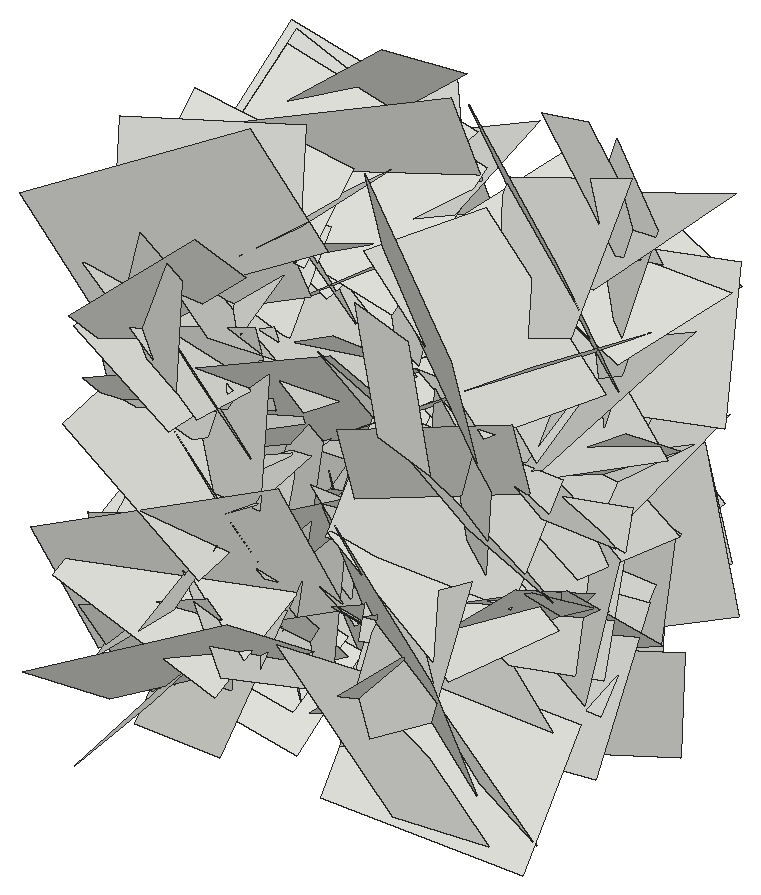
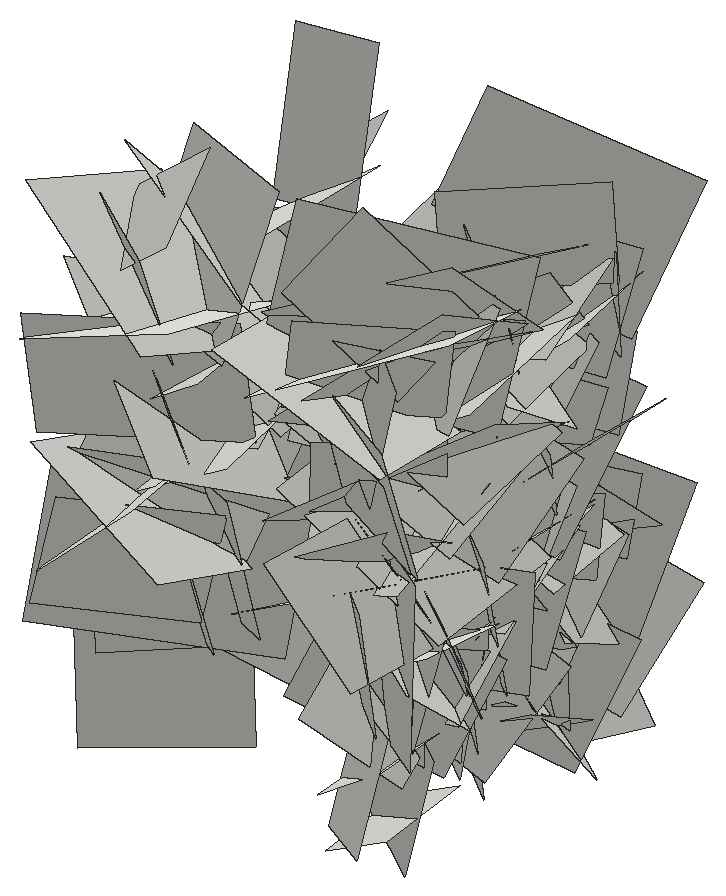
# SketchUp Ruby script. Lengths in inches.
U = 1.inch
M = Sketchup.active_model
def pt(a) = Geom::Point3d.new(a.map { |v| v * U })
def face(e, loops, mat)
  f = e.add_face(loops[0].map { |a| pt(a) })
  loops[1..].each { |l| e.add_face(l.map { |a| pt(a) }).erase! }
  f.material = f.back_material = mat if mat
  f
end
# faces: each face lists its corners as indices into pts; further lists are holes
def faces(e, pts, list, mat = nil) = list.each { |f| face(e, (f[0].is_a?(Array) ? f : [f]).map { |l| l.map { |i| pts[i] } }, mat) }
# xy, xz, yz: faces in a plane at the given z, y or x. An outline is a flat list of corners, or four numbers for a rectangle; further outlines are holes
def ring(l) = l.size == 4 ? [[l[0], l[1]], [l[2], l[1]], [l[2], l[3]], [l[0], l[3]]] : l.each_slice(2).to_a
def flat(e, list, mat, &to3) = list.each { |f| face(e, (f[0].is_a?(Array) ? f : [f]).map { |l| ring(l).map { |u, v| to3.(u, v) } }, mat) }
def xy(e, z, list, mat = nil) = flat(e, list, mat) { |x, y| [x, y, z] }
def xz(e, y, list, mat = nil) = flat(e, list, mat) { |x, z| [x, y, z] }
def yz(e, x, list, mat = nil) = flat(e, list, mat) { |y, z| [x, y, z] }
def lines(e, pts, list) = list.each { |a, b| e.add_line(pt(pts[a]), pt(pts[b])) }
# prism: a flat outline (further loops are holes) pulled along v
def prism(e, loops, v, mat = nil)
  f = face(e, loops, mat); d = Geom::Vector3d.new(v.map { |x| x * U })
  f.pushpull(f.normal.samedirection?(d) ? d.length : -d.length)
end
def box(e, o, s, mat = nil) = prism(e, [[o, [o[0] + s[0], o[1], o[2]], [o[0] + s[0], o[1] + s[1], o[2]], [o[0], o[1] + s[1], o[2]]]], [0, 0, s[2]], mat)
def at(x, y, z, deg = 0) = Geom::Transformation.translation(pt([x, y, z])) * Geom::Transformation.rotation(ORIGIN, Z_AXIS, deg.degrees)
def axes(o, x, y, z) = Geom::Transformation.new([*x, 0, *y, 0, *z, 0, *pt(o).to_a, 1])
def part(name) = M.definitions.add(name)
# library, detail: a bought-in or finely detailed component or shape, given as its bounding box
def library(name, o, s) = part(name).tap { |d| box(d.entities, o, s) }
def detail(e, o, s) = box(e.add_group.entities, o, s)
def put(e, d, t, mat = nil) = e.add_instance(d, t).tap { |i| i.material = mat if mat }
def group(e, t, mat = nil) = e.add_group.tap { |g| g.transformation = t; g.material = mat if mat }.entities
root = M.entities
c1 = part("Component\#6")
p = [[0.01,0,0],[0,3.24,4.54],[4.32,3.24,4.54],[4.33,0,0]]
faces(c1.entities,p,[[0,1,2,3]])
put(root,c1,axes([414.68,153.18,27.99],[0.08911,-1.01671,-0.11332],[0.1646,-0.0997,1.00972],[-1.07181,-0.09984,0.14565]))
put(root,c1,axes([410.71,160.42,26.72],[-0.04031,-0.6417,-0.5437],[0.04231,-0.54502,0.64047],[0.89052,-0.00315,-0.05504]))
put(root,c1,axes([414.68,152.86,32.22],[0.07765,-0.95123,0.12327],[0.10469,0.13045,0.94796],[-1.01133,-0.05954,0.1076]))
put(root,c1,axes([414.68,152.23,36.27],[-0.17612,0.33723,0.58016],[0.03508,0.60107,-0.33991],[-0.71045,-0.05392,-0.16061]))
put(root,c1,axes([410.71,156.02,27.27],[0.01737,0.78195,0.05447],[0.0729,0.05284,-0.77921],[0.82768,-0.02106,0.06749]))
put(root,c1,axes([410.71,151.43,29.49],[-0.01376,0.93036,0.01045],[-0.09599,0.00914,-0.92605],[0.98156,0.01394,-0.09041]))
put(root,c1,axes([410.71,155.63,34.51],[-0.04715,-0.7148,-0.47013],[0.06325,-0.47221,0.71232],[0.90467,-0.00424,-0.0743]))
put(root,c1,axes([414.68,159.35,19.53],[-0.12506,-0.65018,0.20227],[0.00025,0.20525,0.65988],[-0.72178,0.11273,-0.03482]))
put(root,c1,axes([414.68,154.14,39.875],[0.07687,-0.17009,-0.90128],[0.07958,-0.89996,0.17589],[-0.96896,-0.0874,-0.05706]))
put(root,c1,axes([410.71,161.57,34.4],[-0.05292,-0.24359,-0.78611],[0.1523,-0.77804,0.23197],[0.85897,0.12294,-0.08956]))
put(root,c1,axes([410.71,150.44,37.52],[-0.01758,-0.03984,-0.83316],[0.08726,-0.82933,0.03802],[0.87984,0.08145,-0.02042]))
put(root,c1,axes([410.71,152.86,25.21],[0.07237,-0.84668,-0.40971],[-0.16913,-0.41526,0.83156],[0.98259,-0.00911,0.17331]))
put(root,c1,axes([410.71,151.53,22],[-0.08087,0.78957,0.40941],[0.10212,0.41583,-0.78401],[0.93722,0.02282,0.12075]))
put(root,c1,axes([410.71,158.82,28.52],[-0.0834,-0.34729,-0.88838],[0.00654,-0.89156,0.34799],[1.01106,-0.02288,-0.07553]))
put(root,c1,axes([414.68,156.05,22.34],[-0.04217,-0.56806,-0.37659],[-0.07293,-0.37196,0.56834],[-0.71876,0.07107,-0.03557]))
put(root,c1,axes([414.68,160.84,30.26],[-0.09118,-0.56201,-0.30691],[-0.0596,-0.30185,0.56849],[-0.67615,0.1024,-0.00872]))
put(root,c1,axes([410.71,154.61,36.92],[-0.07328,1.03426,0.55463],[-0.26621,0.52968,-1.01904],[1.21518,0.17841,-0.1898]))
put(root,c1,axes([414.68,159.76,21.63],[-0.09665,-0.666,0.12875],[0.03078,0.12595,0.67212],[-0.71837,0.095,0.01147]))
put(root,c1,axes([414.68,147.16,24.1],[0.03025,0.92414,0.23442],[0.23339,0.2218,-0.90118],[-0.98329,0.08108,-0.20669]))
put(root,c1,axes([410.71,157.73,31.39],[-0.13129,-0.92283,0.37392],[0.04334,0.37177,0.93107],[1.05456,-0.13017,0.00829]))
put(root,c1,axes([414.68,159.1875,20.3125],[0.01409,-0.35632,0.80543],[0.16766,0.79339,0.34838],[-0.91839,0.13938,0.07596]))
put(root,c1,axes([414.68,153.92,21.15],[0.0271,-0.2919,0.8704],[0.20523,0.85287,0.28034],[-0.95124,0.17569,0.08528]))
put(root,c1,axes([414.68,149.63,26.39],[0.05575,0.3601,-0.58557],[-0.15834,-0.56726,-0.36226],[-0.71127,0.15451,0.03475]))
put(root,c1,axes([414.68,150.69,21.46],[0.08617,-0.06424,0.73191],[-0.1147,0.7273,0.07585],[-0.77031,-0.11548,0.07058]))
put(root,c1,axes([410.71,152.31,24.83],[0.14132,0.38772,0.61473],[0.11706,0.60692,-0.40674],[0.76145,-0.16526,-0.05156]))
put(root,c1,axes([410.71,150.4,30.92],[0.04252,-0.27759,0.76161],[0.13298,0.75548,0.26875],[0.84891,-0.10444,-0.08025]))
put(root,c1,axes([414.68,156.49,28.09],[-0.01227,0.36562,0.53928],[-0.0952,0.53332,-0.36351],[-0.68404,-0.08079,0.04092]))
put(root,c1,axes([410.71,150.56,37.37],[0.01495,0.72639,-0.4873],[0.06872,-0.48689,-0.7239],[0.92463,0.02444,0.06168]))
put(root,c1,axes([414.68,156.34,37.48],[0.20366,-0.78098,-0.33642],[-0.07649,-0.35863,0.79133],[-0.89812,-0.14656,-0.14368]))
put(root,c1,axes([410.71,156.72,22.08],[-0.00521,-0.94479,0.50901],[-0.17637,0.50353,0.93301],[1.12382,0.07464,0.14878]))
put(root,c1,axes([414.68,158.75,26.14],[-0.12859,0.59437,-0.23179],[0.06253,-0.22448,-0.60651],[-0.67335,-0.13435,-0.01206]))
put(root,c1,axes([410.71,154.45,36.57],[0.07713,0.81709,0.22722],[0.03645,0.22503,-0.82021],[0.89825,-0.07929,0.01378]))
put(root,c1,axes([414.68,149.71,29.1],[-0.04042,0.22115,-0.567],[-0.10046,-0.56334,-0.21335],[-0.63725,0.07479,0.0696]))
put(root,c1,axes([414.68,153.82,25.23],[-0.04726,-0.11023,0.59197],[-0.093,0.58845,0.10297],[-0.63147,-0.07841,-0.05947]))
put(root,c1,axes([410.71,150.92,33.45],[-0.01124,-0.40239,0.85237],[0.02564,0.85203,0.40253],[0.99881,-0.0264,-0.00074]))
put(root,c1,axes([410.71,152.27,30.34],[0.04267,0.47891,-0.74389],[0.05776,-0.74459,-0.47642],[0.93603,0.02411,0.06331]))
put(root,c1,axes([410.71,153.79,24.7],[-0.00565,-0.43188,0.90191],[-0.04751,0.90112,0.43124],[1.05892,0.03812,0.02416]))
put(root,c1,axes([410.71,160.9375,37.33],[0.13153,0.12633,-0.90974],[-0.10231,-0.91113,-0.13969],[0.96819,-0.11344,0.10882]))
put(root,c1,axes([414.68,155.3,36.05],[0.02231,-0.46484,-0.62566],[0.10069,-0.6197,0.4636],[-0.82005,-0.08874,0.0399]))
put(root,c1,axes([410.71,155.99,38.05],[0.0315,0.52335,-0.79271],[-0.01447,-0.79278,-0.52391],[1.00678,-0.02777,0.01727]))
put(root,c1,axes([414.68,150.81,32.67],[0.03105,-0.70657,0.01303],[-0.00041,0.01303,0.70717],[-0.74909,-0.02929,0.00015]))
put(root,c1,axes([410.71,158.65,23.12],[-0.03,-0.65446,0.65644],[0.11713,0.64968,0.65248],[0.97555,-0.09812,-0.05816]))
put(root,c1,axes([414.68,151.89,27.92],[-0.07457,-0.37507,-0.49968],[0.035,-0.50437,0.37394],[-0.66135,0.0156,0.07613]))
put(root,c1,axes([414.68,158.01,30.39],[-0.08038,-0.60995,0.00551],[0.02253,0.00291,0.6143],[-0.64618,0.07598,0.02073]))
put(root,c1,axes([414.68,153.52,29.46],[0.08102,0.00764,-0.81457],[0.10707,-0.81193,0.00187],[-0.85682,-0.10074,-0.07679]))
put(root,c1,axes([410.71,152.65,32.7],[-0.31384,1.21799,0.62272],[-0.13011,0.61092,-1.25326],[1.44417,0.31973,0.02242]))
put(root,c1,axes([410.71,149.65,34.23],[-0.2234,-0.54463,1.08834],[-0.02633,1.10624,0.54877],[1.28976,-0.07175,0.19972]))
put(root,c1,axes([414.68,152.7,33.94],[0.15183,0.13661,-0.74127],[-0.04087,-0.75222,-0.14607],[-0.79793,0.06452,-0.13357]))
put(root,c1,axes([414.68,158.73,27.09],[0.13155,-0.14233,-0.74779],[0.00006,-0.75766,0.14422],[-0.80689,-0.02326,-0.12191]))
put(root,c1,axes([414.68,158.35,30.49],[0.08461,0.81055,-0.03501],[0.12527,-0.04642,-0.80528],[-0.85081,0.07377,-0.12204]))
put(root,c1,axes([410.71,158.66,27.8],[0.19419,0.10037,-0.91545],[-0.10975,-0.92523,-0.12216],[0.97001,-0.12478,0.16945]))
put(root,c1,axes([414.68,156.65,23.33],[-0.01341,0.01203,0.69899],[0.10657,0.69187,-0.01009],[-0.73333,0.10033,-0.01425]))
put(root,c1,axes([410.71,154.96,37.56],[-0.27688,1.1515,0.31839],[0.11464,0.34737,-1.16756],[1.26119,0.22122,0.17603]))
put(root,c1,axes([410.71,152.42,20.54],[-0.05004,-0.6691,0.77955],[0.05919,0.77755,0.67076],[1.08735,-0.07312,-0.00064]))
put(root,c1,axes([414.68,161,38.46],[0.19651,-0.13504,-0.81499],[0.03185,-0.8336,0.14496],[-0.87508,-0.06067,-0.17773]))
put(root,c1,axes([410.71,159.15,23.91],[0.14407,0.13595,-0.90237],[-0.02833,-0.91134,-0.14133],[0.9669,-0.04696,0.13032]))
put(root,c1,axes([410.71,151.25,34.8],[0.16779,0.3958,-0.75565],[0.05631,-0.77163,-0.39305],[0.90246,-0.02545,0.16502]))
put(root,c1,axes([414.68,158.03,24.73],[0.19324,-0.05037,0.89121],[0.15909,0.89838,0.02008],[-0.93272,0.1428,0.18806]))
put(root,c1,axes([410.71,154.4,23.625],[-0.0407,-0.65785,-0.83395],[0.03781,-0.83482,0.65689],[1.12528,0.00426,-0.05223]))
put(root,c1,axes([414.68,157.59,40.82],[0.16311,0.68993,-0.43022],[0.09586,-0.44966,-0.68876],[-0.85651,0.08106,-0.15901]))
put(root,c1,axes([410.71,154.59,24.16],[-0.1724,0.15274,1.09758],[0.17194,1.10067,-0.12914],[1.16199,-0.14021,0.18195]))
put(root,c1,axes([410.71,152.14,28.92],[0.00837,0.82237,-0.50147],[0.16225,-0.49618,-0.8113],[1.00803,0.07304,0.13474]))
put(root,c1,axes([414.68,149.08,38.35],[-0.0057,0.54335,-0.52891],[0.23788,-0.50408,-0.52014],[-0.76776,-0.16022,-0.15723]))
put(root,c1,axes([414.68,157.4,31.875],[0.05779,-0.51798,-0.36432],[0.0587,-0.36037,0.52065],[-0.6687,-0.0764,0.01422]))
put(root,c1,axes([410.71,156.45,32.24],[0.14884,0.843,-0.57449],[-0.06248,-0.57223,-0.85409],[1.07954,-0.14935,0.02978]))
put(root,c1,axes([414.68,160.09,33.87],[0.13785,-0.16653,-0.67513],[0.04892,-0.68326,0.17743],[-0.73546,-0.07666,-0.11474]))
put(root,c1,axes([410.71,156.02,28.65],[-0.0619,-0.85924,0.62732],[0.17366,0.61351,0.85557],[1.11425,-0.14335,-0.09849]))
put(root,c1,axes([410.71,156.69,29.48],[-0.02364,1.01192,0.31394],[0.16386,0.31376,-1.00035],[1.11105,-0.02474,0.15421]))
put(root,c1,axes([410.71,161.68,35.57],[-0.09547,-0.29138,-1.10436],[0.14499,-1.10257,0.27976],[1.20197,0.10985,-0.12146]))
put(root,c1,axes([410.71,147.58,26.68],[0.22766,0.71104,0.67114],[-0.02672,0.69094,-0.72395],[1.03608,-0.13842,-0.16614]))
put(root,c1,axes([410.71,153.43,27.14],[0.15407,-0.97446,-0.01303],[0.08051,-0.00181,0.98239],[1.02988,0.14592,-0.07485]))
put(root,c1,axes([410.71,158.93,27.77],[-0.0679,-1.16178,0.21088],[0.08573,0.20637,1.16154],[1.24867,-0.07734,-0.06828]))
put(root,c1,axes([410.71,160.05,30.35],[-0.12426,0.20575,-1.35522],[-0.11745,-1.35714,-0.19646],[1.44825,-0.0924,-0.13221]))
put(root,c1,axes([410.71,157.84,26.69],[0.16666,-0.37984,-0.88441],[0.10341,-0.88523,0.39754],[1.01503,0.15255,0.10471]))
put(root,c1,axes([410.71,153.58,31.99],[0.17505,-0.32324,-0.90395],[0.10086,-0.9072,0.34179],[1.0126,0.14624,0.12223]))
put(root,c1,axes([410.71,151.45,29.33],[0.11063,1.17252,-0.59491],[-0.28501,-0.56514,-1.16101],[1.36425,-0.21315,-0.19431]))
put(root,c1,axes([410.71,155.57,33.875],[0.13701,-1.11756,0.11199],[-0.07264,0.10468,1.12363],[1.18833,0.13525,0.05577]))
put(root,c1,axes([410.71,156.79,29.67],[0.01777,-0.29003,-1.18393],[-0.05362,-1.18318,0.28913],[1.29096,-0.04516,0.0283]))
put(root,c1,axes([410.71,158.37,30.5],[0.12568,-1.12455,0.31778],[-0.06348,0.31314,1.13049],[1.23707,0.13032,0.02572]))
put(root,c1,axes([410.71,152.25,36.24],[-0.0137,1.21221,-0.26433],[0.01965,-0.26413,-1.21218],[1.31499,0.01657,0.01536]))
put(root,c1,axes([410.71,150.2,21.48],[0.03659,-0.96074,0.6365],[0.08804,0.6372,0.9573],[1.21843,-0.01719,-0.08829]))
put(root,c1,axes([410.71,149.67,23.37],[-0.09539,-0.59855,1.14231],[0.08783,1.14003,0.60389],[1.36418,-0.11525,0.041]))
put(root,c1,axes([410.71,153.92,36.42],[0.14295,0.82362,0.79821],[0.11339,0.79118,-0.83443],[1.21047,-0.17138,-0.0161]))
put(root,c1,axes([410.71,156.14,33.68],[0.06217,-0.55405,1.15944],[0.03014,1.16092,0.55332],[1.36179,-0.0004,-0.06518]))
put(root,c1,axes([410.71,157.5625,26.25],[0.15158,-0.38022,-1.22414],[-0.0526,-1.23246,0.37701],[1.35773,-0.0053,0.15127]))
put(root,c1,axes([410.71,161.74,34.71],[0.1652,-1.10091,-0.16395],[0.26327,-0.12698,1.08875],[1.15009,0.1872,-0.22568]))
put(root,c1,axes([410.71,153.73,28.3],[-0.01858,0.99462,-0.84655],[0.29457,-0.8244,-0.97435],[1.35277,0.19318,0.20054]))
put(root,c1,axes([410.71,153.125,28.17],[-0.03085,-0.9293,0.97672],[0.26234,0.95667,0.91759],[1.40479,-0.19906,-0.14991]))
put(root,c1,axes([410.71,153.14,23.91],[0.18,-1.08552,0.79109],[0.08355,0.80406,1.08641],[1.42134,0.0902,-0.16405]))
put(root,c1,axes([424.49,153.14,23.91],[-0.18,-1.08552,0.79109],[-0.08355,0.80406,1.08641],[-1.42134,0.0902,-0.16405]))
put(root,c1,axes([424.49,153.125,28.17],[0.03085,-0.9293,0.97672],[-0.26234,0.95667,0.91759],[-1.40479,-0.19906,-0.14991]))
put(root,c1,axes([424.49,153.73,28.3],[0.01858,0.99462,-0.84655],[-0.29457,-0.8244,-0.97435],[-1.35277,0.19318,0.20054]))
put(root,c1,axes([424.49,161.74,34.71],[-0.1652,-1.10091,-0.16395],[-0.26327,-0.12698,1.08875],[-1.15009,0.1872,-0.22568]))
put(root,c1,axes([424.49,157.5625,26.25],[-0.15158,-0.38022,-1.22414],[0.0526,-1.23246,0.37701],[-1.35773,-0.0053,0.15127]))
put(root,c1,axes([424.49,156.14,33.68],[-0.06217,-0.55405,1.15944],[-0.03014,1.16092,0.55332],[-1.36179,-0.0004,-0.06518]))
put(root,c1,axes([424.49,153.92,36.42],[-0.14295,0.82362,0.79821],[-0.11339,0.79118,-0.83443],[-1.21047,-0.17138,-0.0161]))
put(root,c1,axes([424.49,149.67,23.37],[0.09539,-0.59855,1.14231],[-0.08783,1.14003,0.60389],[-1.36418,-0.11525,0.041]))
put(root,c1,axes([424.49,150.2,21.48],[-0.03659,-0.96074,0.6365],[-0.08804,0.6372,0.9573],[-1.21843,-0.01719,-0.08829]))
put(root,c1,axes([424.49,152.25,36.24],[0.0137,1.21221,-0.26433],[-0.01965,-0.26413,-1.21218],[-1.31499,0.01657,0.01536]))
put(root,c1,axes([424.49,158.37,30.5],[-0.12568,-1.12455,0.31778],[0.06348,0.31314,1.13049],[-1.23707,0.13032,0.02572]))
put(root,c1,axes([424.49,156.79,29.67],[-0.01777,-0.29003,-1.18393],[0.05362,-1.18318,0.28913],[-1.29096,-0.04516,0.0283]))
put(root,c1,axes([424.49,155.57,33.875],[-0.13701,-1.11756,0.11199],[0.07264,0.10468,1.12363],[-1.18833,0.13525,0.05577]))
put(root,c1,axes([424.49,151.45,29.33],[-0.11063,1.17252,-0.59491],[0.28501,-0.56514,-1.16101],[-1.36425,-0.21315,-0.19431]))
put(root,c1,axes([424.49,153.58,31.99],[-0.17505,-0.32324,-0.90395],[-0.10086,-0.9072,0.34179],[-1.0126,0.14624,0.12223]))
put(root,c1,axes([424.49,157.84,26.69],[-0.16666,-0.37984,-0.88441],[-0.10341,-0.88523,0.39754],[-1.01503,0.15255,0.10471]))
put(root,c1,axes([424.49,160.05,30.35],[0.12426,0.20575,-1.35522],[0.11745,-1.35714,-0.19646],[-1.44825,-0.0924,-0.13221]))
put(root,c1,axes([424.49,158.93,27.77],[0.0679,-1.16178,0.21088],[-0.08573,0.20637,1.16154],[-1.24867,-0.07734,-0.06828]))
put(root,c1,axes([424.49,153.43,27.14],[-0.15407,-0.97446,-0.01303],[-0.08051,-0.00181,0.98239],[-1.02988,0.14592,-0.07485]))
put(root,c1,axes([424.49,147.58,26.68],[-0.22766,0.71104,0.67114],[0.02672,0.69094,-0.72395],[-1.03608,-0.13842,-0.16614]))
put(root,c1,axes([424.49,161.68,35.57],[0.09547,-0.29138,-1.10436],[-0.14499,-1.10257,0.27976],[-1.20197,0.10985,-0.12146]))
put(root,c1,axes([424.49,156.69,29.48],[0.02364,1.01192,0.31394],[-0.16386,0.31376,-1.00035],[-1.11105,-0.02474,0.15421]))
put(root,c1,axes([424.49,156.02,28.65],[0.0619,-0.85924,0.62732],[-0.17366,0.61351,0.85557],[-1.11425,-0.14335,-0.09849]))
put(root,c1,axes([420.52,160.09,33.87],[-0.13785,-0.16653,-0.67513],[-0.04892,-0.68326,0.17743],[0.73546,-0.07666,-0.11474]))
put(root,c1,axes([424.49,156.45,32.24],[-0.14884,0.843,-0.57449],[0.06248,-0.57223,-0.85409],[-1.07954,-0.14935,0.02978]))
put(root,c1,axes([420.52,157.4,31.875],[-0.05779,-0.51798,-0.36432],[-0.0587,-0.36037,0.52065],[0.6687,-0.0764,0.01422]))
put(root,c1,axes([420.52,149.08,38.35],[0.0057,0.54335,-0.52891],[-0.23788,-0.50408,-0.52014],[0.76776,-0.16022,-0.15723]))
put(root,c1,axes([424.49,152.14,28.92],[-0.00837,0.82237,-0.50147],[-0.16225,-0.49618,-0.8113],[-1.00803,0.07304,0.13474]))
put(root,c1,axes([424.49,154.59,24.16],[0.1724,0.15274,1.09758],[-0.17194,1.10067,-0.12914],[-1.16199,-0.14021,0.18195]))
put(root,c1,axes([420.52,157.59,40.82],[-0.16311,0.68993,-0.43022],[-0.09586,-0.44966,-0.68876],[0.85651,0.08106,-0.15901]))
put(root,c1,axes([424.49,154.4,23.625],[0.0407,-0.65785,-0.83395],[-0.03781,-0.83482,0.65689],[-1.12528,0.00426,-0.05223]))
put(root,c1,axes([420.52,158.03,24.73],[-0.19324,-0.05037,0.89121],[-0.15909,0.89838,0.02008],[0.93272,0.1428,0.18806]))
put(root,c1,axes([424.49,151.25,34.8],[-0.16779,0.3958,-0.75565],[-0.05631,-0.77163,-0.39305],[-0.90246,-0.02545,0.16502]))
put(root,c1,axes([424.49,159.15,23.91],[-0.14407,0.13595,-0.90237],[0.02833,-0.91134,-0.14133],[-0.9669,-0.04696,0.13032]))
put(root,c1,axes([420.52,161,38.46],[-0.19651,-0.13504,-0.81499],[-0.03185,-0.8336,0.14496],[0.87508,-0.06067,-0.17773]))
put(root,c1,axes([424.49,152.42,20.54],[0.05004,-0.6691,0.77955],[-0.05919,0.77755,0.67076],[-1.08735,-0.07312,-0.00064]))
put(root,c1,axes([424.49,154.96,37.56],[0.27688,1.1515,0.31839],[-0.11464,0.34737,-1.16756],[-1.26119,0.22122,0.17603]))
put(root,c1,axes([420.52,156.65,23.33],[0.01341,0.01203,0.69899],[-0.10657,0.69187,-0.01009],[0.73333,0.10033,-0.01425]))
put(root,c1,axes([424.49,158.66,27.8],[-0.19419,0.10037,-0.91545],[0.10975,-0.92523,-0.12216],[-0.97001,-0.12478,0.16945]))
put(root,c1,axes([420.52,158.35,30.49],[-0.08461,0.81055,-0.03501],[-0.12527,-0.04642,-0.80528],[0.85081,0.07377,-0.12204]))
put(root,c1,axes([420.52,158.73,27.09],[-0.13155,-0.14233,-0.74779],[-0.00006,-0.75766,0.14422],[0.80689,-0.02326,-0.12191]))
put(root,c1,axes([420.52,152.7,33.94],[-0.15183,0.13661,-0.74127],[0.04087,-0.75222,-0.14607],[0.79793,0.06452,-0.13357]))
put(root,c1,axes([424.49,149.65,34.23],[0.2234,-0.54463,1.08834],[0.02633,1.10624,0.54877],[-1.28976,-0.07175,0.19972]))
put(root,c1,axes([424.49,152.65,32.7],[0.31384,1.21799,0.62272],[0.13011,0.61092,-1.25326],[-1.44417,0.31973,0.02242]))
